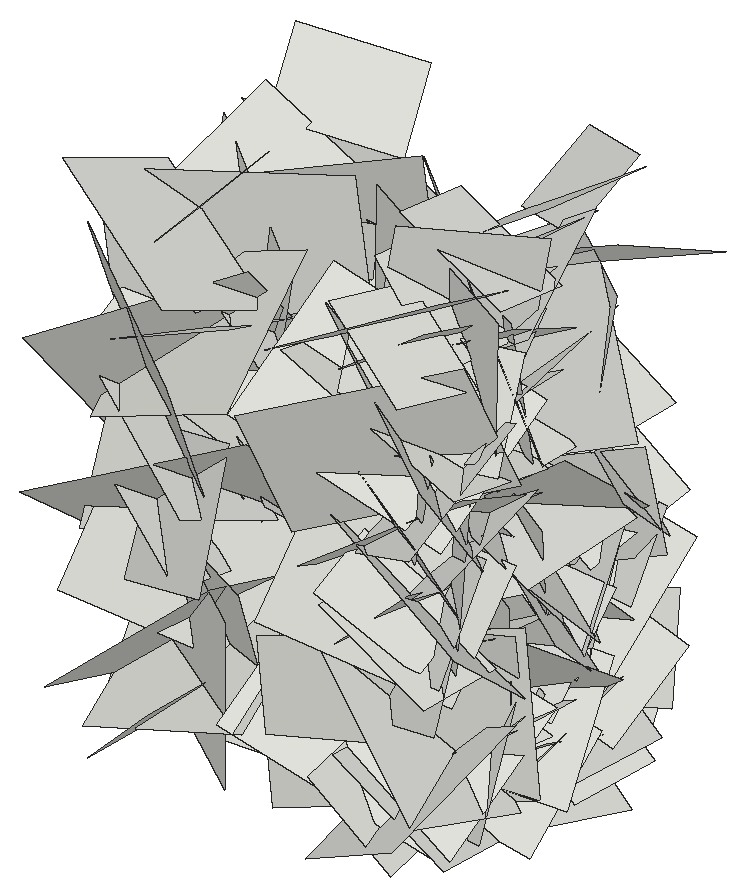
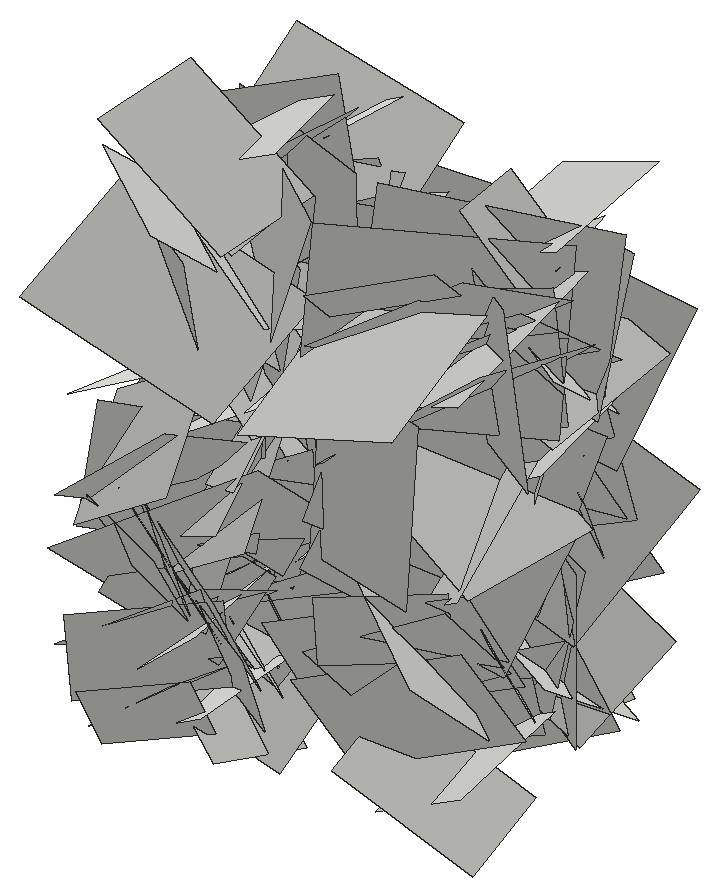
# SketchUp Ruby script. Lengths in inches.
U = 1.inch
M = Sketchup.active_model
def pt(a) = Geom::Point3d.new(a.map { |v| v * U })
def face(e, loops, mat)
  f = e.add_face(loops[0].map { |a| pt(a) })
  loops[1..].each { |l| e.add_face(l.map { |a| pt(a) }).erase! }
  f.material = f.back_material = mat if mat
  f
end
# faces: each face lists its corners as indices into pts; further lists are holes
def faces(e, pts, list, mat = nil) = list.each { |f| face(e, (f[0].is_a?(Array) ? f : [f]).map { |l| l.map { |i| pts[i] } }, mat) }
# xy, xz, yz: faces in a plane at the given z, y or x. An outline is a flat list of corners, or four numbers for a rectangle; further outlines are holes
def ring(l) = l.size == 4 ? [[l[0], l[1]], [l[2], l[1]], [l[2], l[3]], [l[0], l[3]]] : l.each_slice(2).to_a
def flat(e, list, mat, &to3) = list.each { |f| face(e, (f[0].is_a?(Array) ? f : [f]).map { |l| ring(l).map { |u, v| to3.(u, v) } }, mat) }
def xy(e, z, list, mat = nil) = flat(e, list, mat) { |x, y| [x, y, z] }
def xz(e, y, list, mat = nil) = flat(e, list, mat) { |x, z| [x, y, z] }
def yz(e, x, list, mat = nil) = flat(e, list, mat) { |y, z| [x, y, z] }
def lines(e, pts, list) = list.each { |a, b| e.add_line(pt(pts[a]), pt(pts[b])) }
# prism: a flat outline (further loops are holes) pulled along v
def prism(e, loops, v, mat = nil)
  f = face(e, loops, mat); d = Geom::Vector3d.new(v.map { |x| x * U })
  f.pushpull(f.normal.samedirection?(d) ? d.length : -d.length)
end
def box(e, o, s, mat = nil) = prism(e, [[o, [o[0] + s[0], o[1], o[2]], [o[0] + s[0], o[1] + s[1], o[2]], [o[0], o[1] + s[1], o[2]]]], [0, 0, s[2]], mat)
def at(x, y, z, deg = 0) = Geom::Transformation.translation(pt([x, y, z])) * Geom::Transformation.rotation(ORIGIN, Z_AXIS, deg.degrees)
def axes(o, x, y, z) = Geom::Transformation.new([*x, 0, *y, 0, *z, 0, *pt(o).to_a, 1])
def part(name) = M.definitions.add(name)
# library, detail: a bought-in or finely detailed component or shape, given as its bounding box
def library(name, o, s) = part(name).tap { |d| box(d.entities, o, s) }
def detail(e, o, s) = box(e.add_group.entities, o, s)
def put(e, d, t, mat = nil) = e.add_instance(d, t).tap { |i| i.material = mat if mat }
def group(e, t, mat = nil) = e.add_group.tap { |g| g.transformation = t; g.material = mat if mat }.entities
root = M.entities
c1 = part("Component\#6")
p = [[0.01,0,0],[0,3.24,4.54],[4.32,3.24,4.54],[4.33,0,0]]
faces(c1.entities,p,[[0,1,2,3]])
put(root,c1,axes([400.91,138.81,37.71],[-0.08326,0.50336,-1.07522],[-0.02589,-1.07803,-0.50289],[1.25818,0.01113,-0.0815]))
put(root,c1,axes([414.68,138.81,37.71],[0.08326,0.50336,-1.07522],[0.02589,-1.07803,-0.50289],[-1.25818,0.01113,-0.0815]))
put(root,c1,axes([410.71,136.62,23.89],[-0.08859,0.63974,0.04756],[-0.12242,0.03217,-0.63572],[0.66888,0.09062,-0.11005]))
put(root,c1,axes([404.88,136.62,23.89],[0.08859,0.63974,0.04756],[0.12242,0.03217,-0.63572],[-0.66888,0.09062,-0.11005]))
put(root,c1,axes([414.68,139.47,36.72],[-0.15825,-0.66033,0.08813],[-0.02764,0.09604,0.67542],[-0.70562,0.14433,-0.04622]))
put(root,c1,axes([414.68,138.53,29.67],[-0.03677,-0.4198,0.69058],[-0.10131,0.68849,0.41374],[-0.85065,-0.06385,-0.07912]))
put(root,c1,axes([410.71,136.92,29.78],[0.03864,0.57092,0.32429],[-0.05823,0.3263,-0.56829],[0.69355,-0.00442,-0.06578]))
put(root,c1,axes([410.71,137.14,29.31],[0.00249,0.75761,-0.01469],[0.08098,-0.01485,-0.75375],[0.79913,-0.00085,0.07643]))
put(root,c1,axes([400.91,137.65,40.3125],[0.15365,0.92766,-0.3555],[0.07441,-0.36793,-0.93147],[1.05042,-0.10963,0.11798]))
put(root,c1,axes([414.68,137.65,40.3125],[-0.15365,0.92766,-0.3555],[-0.07441,-0.36793,-0.93147],[-1.05042,-0.10963,0.11798]))
put(root,c1,axes([400.91,141.2,30.22],[0.14348,-0.5033,-0.91823],[0.06175,-0.92081,0.51331],[1.10823,0.11647,0.09028]))
put(root,c1,axes([414.68,141.2,30.22],[-0.14348,-0.5033,-0.91823],[-0.06175,-0.92081,0.51331],[-1.10823,0.11647,0.09028]))
put(root,c1,axes([414.68,135.48,23.28],[0.21581,1.04519,0.5846],[0.09636,0.57779,-1.06467],[-1.26577,0.22219,0.01862]))
put(root,c1,axes([410.71,140.39,26.94],[-0.03872,-0.62994,0.14227],[-0.11345,0.14643,0.62088],[0.67508,-0.01152,0.1125]))
put(root,c1,axes([404.88,140.39,26.94],[0.03872,-0.62994,0.14227],[0.11345,0.14643,0.62088],[-0.67508,-0.01152,0.1125]))
put(root,c1,axes([410.71,141.16,33.73],[0.01034,-0.20439,-0.70125],[-0.11317,-0.69418,0.20085],[0.76594,-0.09981,0.03914]))
put(root,c1,axes([400.91,139.67,30.68],[-0.09112,-0.77438,0.96294],[-0.03313,0.96632,0.77431],[1.3094,-0.02944,0.0866]))
put(root,c1,axes([414.68,139.67,30.68],[0.09112,-0.77438,0.96294],[0.03313,0.96632,0.77431],[-1.3094,-0.02944,0.0866]))
put(root,c1,axes([410.71,137.77,24.11],[-0.1419,0.78136,-0.16109],[0.04598,-0.15597,-0.79258],[0.84441,0.13979,0.01609]))
put(root,c1,axes([400.91,141.59,27.99],[-0.06396,0.08339,-1.32201],[-0.02487,-1.32324,-0.0824],[1.4039,-0.01964,-0.06169]))
put(root,c1,axes([414.68,141.59,27.99],[0.06396,0.08339,-1.32201],[0.02487,-1.32324,-0.0824],[-1.4039,-0.01964,-0.06169]))
put(root,c1,axes([410.71,137.53,34.5],[-0.08019,0.3809,0.76753],[0.04804,0.77121,-0.37826],[0.90698,-0.00717,0.08789]))
put(root,c1,axes([400.91,142.63,35.02],[0.11092,-0.98462,-0.77371],[0.1183,-0.76598,0.98988],[1.32209,0.15114,-0.02366]))
put(root,c1,axes([414.68,142.63,35.02],[-0.11092,-0.98462,-0.77371],[-0.1183,-0.76598,0.98988],[-1.32209,0.15114,-0.02366]))
put(root,c1,axes([400.91,141.41,21.99],[0.04242,-1.10503,0.33762],[-0.18816,0.32793,1.09436],[1.21025,0.08972,0.15831]))
put(root,c1,axes([414.68,141.41,21.99],[-0.04242,-1.10503,0.33762],[0.18816,0.32793,1.09436],[-1.21025,0.08972,0.15831]))
put(root,c1,axes([414.68,136.3,32.46],[0.17238,0.91042,0.71253],[0.07022,0.71102,-0.92361],[-1.22345,0.16908,0.04738]))
put(root,c1,axes([404.88,141.05,35.76],[0.06877,-0.60814,0.14272],[0.00885,0.14432,0.61116],[-0.66208,-0.06124,0.02299]))
put(root,c1,axes([410.71,141.05,35.76],[-0.06877,-0.60814,0.14272],[-0.00885,0.14432,0.61116],[0.66208,-0.06124,0.02299]))
put(root,c1,axes([400.91,143.09,24.72],[0.05768,-1.1082,-0.74759],[0.23067,-0.73089,1.09928],[1.3981,0.16631,-0.15052]))
put(root,c1,axes([414.68,143.09,24.72],[-0.05768,-1.1082,-0.74759],[-0.23067,-0.73089,1.09928],[-1.3981,0.16631,-0.15052]))
put(root,c1,axes([414.68,137.68,27.62],[-0.00267,0.49736,0.77514],[-0.05686,0.77375,-0.49665],[-0.97459,-0.04651,0.02685]))
put(root,c1,axes([400.91,138.75,33.42],[0.07987,0.93748,-0.3836],[-0.04246,-0.3816,-0.94046],[1.07286,-0.0849,-0.00867]))
put(root,c1,axes([414.68,138.75,33.42],[-0.07987,0.93748,-0.3836],[0.04246,-0.3816,-0.94046],[-1.07286,-0.0849,-0.00867]))
put(root,c1,axes([400.91,141.71,25.57],[-0.24627,-1.07768,0.84944],[0.21085,0.82598,1.10232],[1.43917,-0.30542,-0.01615]))
put(root,c1,axes([414.68,141.71,25.57],[0.24627,-1.07768,0.84944],[-0.21085,0.82598,1.10232],[-1.43917,-0.30542,-0.01615]))
put(root,c1,axes([400.91,142.6875,32.73],[-0.11413,-1.14483,0.29443],[0.2702,0.26621,1.12831],[1.22353,-0.16558,-0.2217]))
put(root,c1,axes([414.68,142.6875,32.73],[0.11413,-1.14483,0.29443],[-0.2702,0.26621,1.12831],[-1.22353,-0.16558,-0.2217]))
put(root,c1,axes([400.91,141.15,27.9],[0.10356,0.25866,-1.08582],[0.18317,-1.08033,-0.24181],[1.16891,0.14638,0.13409]))
put(root,c1,axes([414.68,141.15,27.9],[-0.10356,0.25866,-1.08582],[-0.18317,-1.08033,-0.24181],[-1.16891,0.14638,0.13409]))
put(root,c1,axes([400.91,137.42,26.21],[0.14568,0.69276,1.17725],[0.03045,1.18146,-0.69859],[1.44759,-0.09457,-0.10377]))
put(root,c1,axes([414.68,137.42,26.21],[-0.14568,0.69276,1.17725],[-0.03045,1.18146,-0.69859],[-1.44759,-0.09457,-0.10377]))
put(root,c1,axes([414.68,137.85,30.84],[0.06669,0.91948,0.38333],[0.06841,0.37952,-0.92095],[-1.05374,0.08283,-0.03553]))
put(root,c1,axes([410.71,143.53,22.21],[-0.15224,-0.84766,-0.36991],[-0.10957,-0.35729,0.85887],[0.97421,-0.17265,0.03879]))
put(root,c1,axes([410.71,139.71,39.61],[0.08624,0.67106,-0.00672],[-0.16105,0.01183,-0.6586],[0.69289,-0.08077,-0.15225]))
put(root,c1,axes([404.88,139.71,39.61],[-0.08624,0.67106,-0.00672],[0.16105,0.01183,-0.6586],[-0.69289,-0.08077,-0.15225]))
put(root,c1,axes([400.91,138.43,27.8],[0.10648,0.28124,1.16655],[-0.16097,1.1642,-0.2676],[1.26174,0.12479,-0.13259]))
put(root,c1,axes([414.68,138.43,27.8],[-0.10648,0.28124,1.16655],[0.16097,1.1642,-0.2676],[-1.26174,0.12479,-0.13259]))
put(root,c1,axes([410.71,139.84,37.375],[0.13047,0.02824,0.77],[-0.11824,0.77221,-0.01049],[0.80815,0.10842,-0.12584]))
put(root,c1,axes([400.91,140.25,33.3],[-0.10371,-0.10781,1.29757],[0.22808,1.282,0.12274],[1.36119,-0.22303,0.07829]))
put(root,c1,axes([414.68,140.25,33.3],[0.10371,-0.10781,1.29757],[-0.22808,1.282,0.12274],[-1.36119,-0.22303,0.07829]))
put(root,c1,axes([400.91,139.49,21.74],[0.04906,0.46783,0.90513],[0.0041,0.90598,-0.46846],[1.08001,-0.02469,-0.03934]))
put(root,c1,axes([414.68,139.49,21.74],[-0.04906,0.46783,0.90513],[-0.0041,0.90598,-0.46846],[-1.08001,-0.02469,-0.03934]))
put(root,c1,axes([410.71,142.28,27.34],[-0.09885,-0.42767,0.49172],[0.03253,0.4933,0.43487],[0.69002,-0.08452,0.04994]))
put(root,c1,axes([404.88,142.28,27.34],[0.09885,-0.42767,0.49172],[-0.03253,0.4933,0.43487],[-0.69002,-0.08452,0.04994]))
put(root,c1,axes([410.71,143.38,25.93],[-0.00088,-0.66729,0.07011],[0.1194,0.06898,0.65784],[0.70113,-0.01259,-0.11194]))
put(root,c1,axes([400.91,139.39,34.34],[0.15089,0.92592,0.71699],[0.08883,0.71236,-0.93659],[1.23815,-0.16395,-0.02018]))
put(root,c1,axes([414.68,139.39,34.34],[-0.15089,0.92592,0.71699],[-0.08883,0.71236,-0.93659],[-1.23815,-0.16395,-0.02018]))
put(root,c1,axes([410.71,144.18,33.46],[-0.08879,-0.56105,-0.39599],[0.0694,-0.40364,0.55803],[0.72461,-0.03009,-0.10197]))
put(root,c1,axes([410.71,144.6,22.65],[-0.17478,-0.82558,-0.09028],[0.09417,-0.10904,0.83495],[0.87528,-0.15312,-0.10786]))
put(root,c1,axes([414.68,145.12,23.07],[0.0526,-0.82286,-0.58821],[-0.0059,-0.58914,0.82367],[-1.07215,-0.03713,-0.03339]))
put(root,c1,axes([414.68,145.6875,25.3],[0.21495,-0.77208,-0.77151],[0.06755,-0.77499,0.79232],[-1.15499,-0.18901,-0.09724]))
put(root,c1,axes([410.71,140.84,40.56],[-0.05261,0.712,-0.12967],[0.10362,-0.12219,-0.70833],[0.7601,0.06594,0.08758]))
put(root,c1,axes([410.71,144.73,33.27],[-0.16555,-0.76551,-0.15352],[0.02389,-0.16091,0.77946],[0.82725,-0.14855,-0.05323]))
put(root,c1,axes([410.71,140.76,35.5625],[0.0095,0.80566,-0.00603],[-0.04784,-0.00552,-0.80445],[0.85268,-0.00929,-0.04507]))
put(root,c1,axes([410.71,143.64,28.51],[0.01569,-0.00258,-0.72773],[0.02057,-0.72762,0.00297],[0.77112,0.01947,0.01473]))
put(root,c1,axes([400.91,141,38.04],[0.14868,1.2474,-0.57055],[0.09146,-0.58042,-1.24775],[1.45112,-0.09122,0.1371]))
put(root,c1,axes([414.68,141,38.04],[-0.14868,1.2474,-0.57055],[-0.09146,-0.58042,-1.24775],[-1.45112,-0.09122,0.1371]))
put(root,c1,axes([414.68,141.61,27.46],[0.15544,0.8369,-0.58263],[0.03072,-0.5918,-0.84279],[-1.08048,0.10358,-0.10778]))
put(root,c1,axes([410.71,142.8,24.59],[-0.06246,-0.31977,0.5346],[0.03506,0.53462,0.32343],[0.65938,-0.05871,0.03344]))
put(root,c1,axes([404.88,142.8,24.59],[0.06246,-0.31977,0.5346],[-0.03506,0.53462,0.32343],[-0.65938,-0.05871,0.03344]))
put(root,c1,axes([400.91,145.76,27.48],[0.11303,-0.66031,-0.96553],[-0.02355,-0.9705,0.66125],[1.23968,0.04176,0.1006]))
put(root,c1,axes([414.68,145.76,27.48],[-0.11303,-0.66031,-0.96553],[0.02355,-0.9705,0.66125],[-1.23968,0.04176,0.1006]))
put(root,c1,axes([400.91,145.05,38.54],[-0.26561,0.06521,-1.32838],[-0.06869,-1.35074,-0.05408],[1.4081,-0.05359,-0.25321]))
put(root,c1,axes([414.68,145.05,38.54],[0.26561,0.06521,-1.32838],[0.06869,-1.35074,-0.05408],[-1.4081,-0.05359,-0.25321]))
put(root,c1,axes([410.71,144.97,35.07],[-0.07722,-0.5315,-0.34657],[-0.05738,-0.34237,0.53643],[0.67013,-0.09056,0.006]))
put(root,c1,axes([404.88,144.97,35.07],[0.07722,-0.5315,-0.34657],[0.05738,-0.34237,0.53643],[-0.67013,-0.09056,0.006]))
put(root,c1,axes([414.68,144.76,23.61],[-0.10873,-0.7568,0.02149],[0.01122,0.02025,0.76368],[-0.80245,0.10283,0.00777]))
put(root,c1,axes([400.91,141.99,33.2],[0.15631,-0.03731,1.01998],[0.08418,1.02787,0.02612],[1.07863,-0.07482,-0.14985]))
put(root,c1,axes([414.68,141.99,33.2],[-0.15631,-0.03731,1.01998],[-0.08418,1.02787,0.02612],[-1.07863,-0.07482,-0.14985]))
put(root,c1,axes([410.71,144.05,31.85],[-0.11078,0.17753,-0.74918],[0.12323,-0.74375,-0.19246],[0.80677,0.13798,-0.07348]))
put(root,c1,axes([410.71,145.49,24.46],[-0.14807,-0.32942,-0.64401],[0.00647,-0.65643,0.33444],[0.76675,-0.05808,-0.12719]))
put(root,c1,axes([404.88,145.49,24.46],[0.14807,-0.32942,-0.64401],[-0.00647,-0.65643,0.33444],[-0.76675,-0.05808,-0.12719]))
put(root,c1,axes([400.91,143.42,27.33],[0.08667,-0.86973,1.01008],[-0.23887,0.9884,0.86929],[1.39256,0.22367,0.08625]))
put(root,c1,axes([414.68,143.42,27.33],[-0.08667,-0.86973,1.01008],[0.23887,0.9884,0.86929],[-1.39256,0.22367,0.08625]))
put(root,c1,axes([400.91,142.58,23.75],[0.11698,0.88265,-0.34817],[-0.00423,-0.35009,-0.88876],[1.00576,-0.10414,0.03675]))
put(root,c1,axes([414.68,142.58,23.75],[-0.11698,0.88265,-0.34817],[0.00423,-0.35009,-0.88876],[-1.00576,-0.10414,0.03675]))
put(root,c1,axes([400.91,140.69,35.43],[0.02714,1.22478,0.26938],[-0.1382,0.27058,-1.21783],[1.3221,0.00314,-0.13283]))
put(root,c1,axes([414.68,140.69,35.43],[-0.02714,1.22478,0.26938],[0.1382,0.27058,-1.21783],[-1.3221,0.00314,-0.13283]))
put(root,c1,axes([400.91,146.73,29.36],[-0.09029,-1.26195,0.03468],[0.03892,0.03227,1.26436],[1.33761,-0.08612,-0.03444]))
put(root,c1,axes([414.68,146.73,29.36],[0.09029,-1.26195,0.03468],[-0.03892,0.03227,1.26436],[-1.33761,-0.08612,-0.03444]))
put(root,c1,axes([400.91,143.41,32.67],[-0.00295,0.89075,-0.72818],[-0.15415,-0.72261,-0.88339],[1.20976,-0.08991,-0.11434]))
put(root,c1,axes([414.68,143.41,32.67],[0.00295,0.89075,-0.72818],[0.15415,-0.72261,-0.88339],[-1.20976,-0.08991,-0.11434]))
put(root,c1,axes([400.91,142.42,32.89],[0.18672,-0.42722,1.28431],[-0.1337,1.28432,0.44452],[1.42847,0.17605,-0.12627]))
put(root,c1,axes([414.68,142.42,32.89],[-0.18672,-0.42722,1.28431],[0.1337,1.28432,0.44452],[-1.42847,0.17605,-0.12627]))
put(root,c1,axes([400.91,141.72,37.36],[0.19445,0.97106,0.50245],[-0.00165,0.50971,-0.98451],[1.15895,-0.1622,-0.0857]))
put(root,c1,axes([414.68,141.72,37.36],[-0.19445,0.97106,0.50245],[0.00165,0.50971,-0.98451],[-1.15895,-0.1622,-0.0857]))
put(root,c1,axes([414.68,145.42,24.52],[0.2647,-0.88765,0.75819],[0.01358,0.77738,0.90589],[-1.23735,-0.18136,0.17214]))
put(root,c1,axes([414.68,141.63,23.18],[0.01995,1.00092,0.30572],[0.13829,0.30114,-0.99396],[-1.10071,0.05598,-0.11933]))
put(root,c1,axes([410.71,145.72,37.21],[0.0202,-0.65006,0.07365],[-0.02062,0.07308,0.65011],[0.69316,0.02112,0.01719]))
put(root,c1,axes([400.91,145.04,25.97],[-0.0145,-0.85349,0.83598],[-0.13626,0.83223,0.84756],[1.25903,0.08024,0.10136]))
put(root,c1,axes([414.68,145.04,25.97],[0.0145,-0.85349,0.83598],[0.13626,0.83223,0.84756],[-1.25903,0.08024,0.10136]))
put(root,c1,axes([414.68,142.67,41.25],[0.05619,0.9574,-0.08237],[-0.00834,-0.08206,-0.95886],[-1.01856,0.05349,0.00331]))
put(root,c1,axes([400.91,146.5,19.86],[0.14062,-0.87102,0.18651],[0.03259,0.19294,0.87915],[0.94365,0.12313,-0.05815]))
put(root,c1,axes([414.68,146.5,19.86],[-0.14062,-0.87102,0.18651],[-0.03259,0.19294,0.87915],[-0.94365,0.12313,-0.05815]))
put(root,c1,axes([410.71,145.6,27.28],[0.00806,0.29423,-0.56577],[0.12293,-0.55701,-0.28812],[0.6647,0.09945,0.06014]))
put(root,c1,axes([414.68,147.86,21.63],[0.08807,-1.00346,0.13322],[0.11481,0.14172,0.99989],[-1.06685,-0.06759,0.1186]))
put(root,c1,axes([410.71,146.3,23.53],[-0.0913,-0.50535,0.50896],[0.05568,0.5068,0.51209],[0.75823,-0.09807,0.02368]))
put(root,c1,axes([400.91,143.97,23.32],[0.18437,0.48358,0.83906],[0.16998,0.82633,-0.50949],[1.01237,-0.22682,-0.06726]))
put(root,c1,axes([414.68,143.97,23.32],[-0.18437,0.48358,0.83906],[-0.16998,0.82633,-0.50949],[-1.01237,-0.22682,-0.06726]))
put(root,c1,axes([414.68,147.08,31.53],[0.0186,0.21399,-0.90436],[0.04027,-0.90393,-0.21315],[-0.98427,-0.03294,-0.02581]))
put(root,c1,axes([400.91,149.48,27.53],[0.05839,-0.93868,-0.8352],[-0.07486,-0.83699,0.93604],[1.32974,-0.0059,0.08937]))
put(root,c1,axes([414.68,149.48,27.53],[-0.05839,-0.93868,-0.8352],[0.07486,-0.83699,0.93604],[-1.32974,-0.0059,0.08937]))
put(root,c1,axes([410.71,144.98,23.12],[0.11015,0.70988,0.06167],[-0.04855,0.06885,-0.71532],[0.75374,-0.09931,-0.05509]))
put(root,c1,axes([400.91,144,25.2],[0.04504,0.58566,0.95802],[0.11757,0.95183,-0.5868],[1.18441,-0.11675,0.02182]))
put(root,c1,axes([414.68,144,25.2],[-0.04504,0.58566,0.95802],[-0.11757,0.95183,-0.5868],[-1.18441,-0.11675,0.02182]))
put(root,c1,axes([400.91,144.65,25.96],[0.15377,0.53431,0.65108],[0.06081,0.65286,-0.54856],[0.89071,-0.13681,-0.07495]))
put(root,c1,axes([414.68,144.65,25.96],[-0.15377,0.53431,0.65108],[-0.06081,0.65286,-0.54856],[-0.89071,-0.13681,-0.07495]))
put(root,c1,axes([414.68,149.13,24.11],[0.03147,-0.85153,-0.39996],[0.02133,-0.3995,0.85202],[-0.997,-0.03542,0.00561]))
put(root,c1,axes([414.68,144.71,33.13],[0.16995,0.04512,1.05289],[0.00982,1.0649,-0.04705],[-1.11704,0.01623,0.15977]))
put(root,c1,axes([414.68,148.52,32.35],[-0.08011,-0.79067,-0.06214],[-0.07476,-0.05548,0.79163],[-0.83736,0.0806,-0.06473]))
put(root,c1,axes([414.68,149.17,29.19],[-0.22051,-0.77582,-0.34275],[0.07369,-0.36732,0.78924],[-0.89602,0.16072,0.14925]))
put(root,c1,axes([410.71,149.56,39.6],[-0.17317,-0.50739,-0.45031],[0.03865,-0.46908,0.51531],[0.71806,-0.09712,-0.13634]))
put(root,c1,axes([404.88,149.56,39.6],[0.17317,-0.50739,-0.45031],[-0.03865,-0.46908,0.51531],[-0.71806,-0.09712,-0.13634]))
put(root,c1,axes([410.71,149.12,29.1],[-0.10824,-0.19319,-0.65872],[-0.02698,-0.66445,0.19881],[0.72715,-0.05341,-0.09068]))
put(root,c1,axes([404.88,149.12,29.1],[0.10824,-0.19319,-0.65872],[0.02698,-0.66445,0.19881],[-0.72715,-0.05341,-0.09068]))
put(root,c1,axes([410.71,146.7,34.04],[-0.22474,0.77203,-0.6543],[-0.03576,-0.67353,-0.78378],[1.07212,0.13937,-0.1633]))
put(root,c1,axes([410.71,145.7,22.51],[-0.08358,0.19729,0.79599],[-0.0899,0.79341,-0.20506],[0.86462,0.10156,0.05562]))
put(root,c1,axes([400.91,145.83,38.68],[-0.04371,1.09164,-0.51046],[0.28885,-0.48908,-1.06793],[1.24431,0.15188,0.22998]))
put(root,c1,axes([414.68,145.83,38.68],[0.04371,1.09164,-0.51046],[-0.28885,-0.48908,-1.06793],[-1.24431,0.15188,0.22998]))
put(root,c1,axes([410.71,146.45,21.25],[-0.00375,0.2874,0.54008],[0.0654,0.5375,-0.28562],[0.64519,-0.05282,0.03209]))
put(root,c1,axes([410.71,149.44,28.46],[-0.01637,-0.35652,-0.61871],[0.18604,-0.60176,0.34238],[0.7337,0.14463,-0.10062]))
put(root,c1,axes([400.91,149.09,36.34],[-0.1737,0.35213,-1.24285],[0.08,-1.24806,-0.36356],[1.36694,0.11779,-0.13666]))
